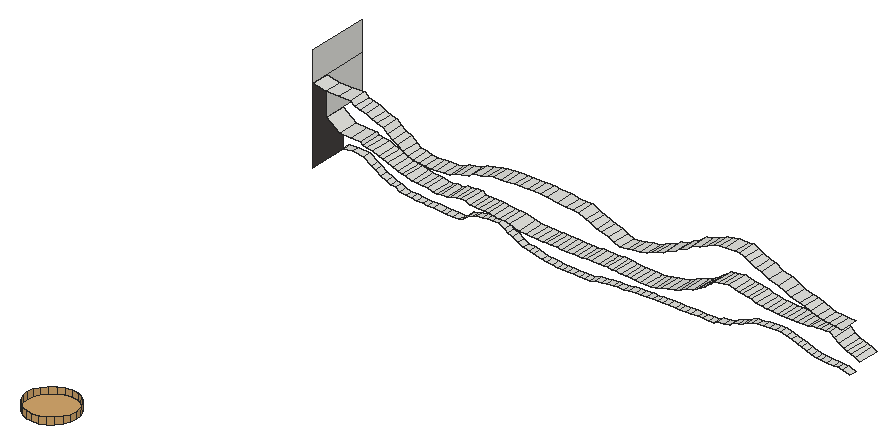
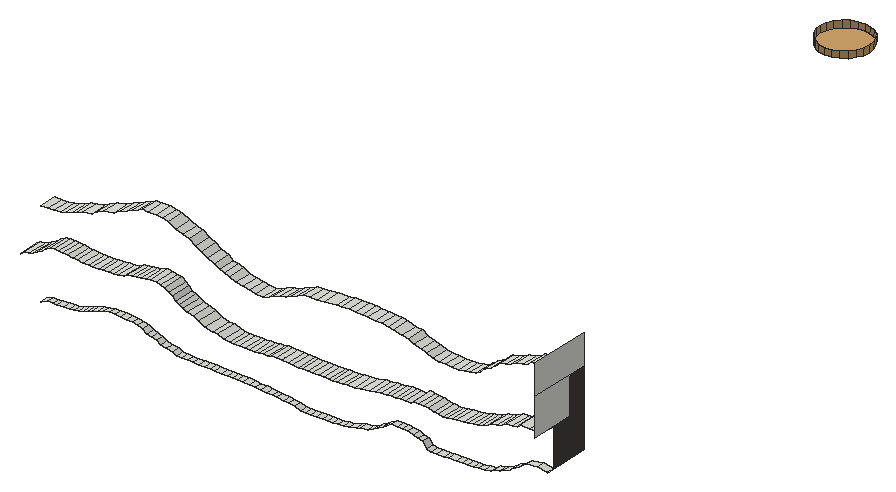
# SketchUp Ruby script. Lengths in inches.
U = 1.inch
M = Sketchup.active_model
def pt(a) = Geom::Point3d.new(a.map { |v| v * U })
def face(e, loops, mat)
  f = e.add_face(loops[0].map { |a| pt(a) })
  loops[1..].each { |l| e.add_face(l.map { |a| pt(a) }).erase! }
  f.material = f.back_material = mat if mat
  f
end
# faces: each face lists its corners as indices into pts; further lists are holes
def faces(e, pts, list, mat = nil) = list.each { |f| face(e, (f[0].is_a?(Array) ? f : [f]).map { |l| l.map { |i| pts[i] } }, mat) }
# xy, xz, yz: faces in a plane at the given z, y or x. An outline is a flat list of corners, or four numbers for a rectangle; further outlines are holes
def ring(l) = l.size == 4 ? [[l[0], l[1]], [l[2], l[1]], [l[2], l[3]], [l[0], l[3]]] : l.each_slice(2).to_a
def flat(e, list, mat, &to3) = list.each { |f| face(e, (f[0].is_a?(Array) ? f : [f]).map { |l| ring(l).map { |u, v| to3.(u, v) } }, mat) }
def xy(e, z, list, mat = nil) = flat(e, list, mat) { |x, y| [x, y, z] }
def xz(e, y, list, mat = nil) = flat(e, list, mat) { |x, z| [x, y, z] }
def yz(e, x, list, mat = nil) = flat(e, list, mat) { |y, z| [x, y, z] }
def lines(e, pts, list) = list.each { |a, b| e.add_line(pt(pts[a]), pt(pts[b])) }
# prism: a flat outline (further loops are holes) pulled along v
def prism(e, loops, v, mat = nil)
  f = face(e, loops, mat); d = Geom::Vector3d.new(v.map { |x| x * U })
  f.pushpull(f.normal.samedirection?(d) ? d.length : -d.length)
end
def box(e, o, s, mat = nil) = prism(e, [[o, [o[0] + s[0], o[1], o[2]], [o[0] + s[0], o[1] + s[1], o[2]], [o[0], o[1] + s[1], o[2]]]], [0, 0, s[2]], mat)
def at(x, y, z, deg = 0) = Geom::Transformation.translation(pt([x, y, z])) * Geom::Transformation.rotation(ORIGIN, Z_AXIS, deg.degrees)
def axes(o, x, y, z) = Geom::Transformation.new([*x, 0, *y, 0, *z, 0, *pt(o).to_a, 1])
def part(name) = M.definitions.add(name)
# library, detail: a bought-in or finely detailed component or shape, given as its bounding box
def library(name, o, s) = part(name).tap { |d| box(d.entities, o, s) }
def detail(e, o, s) = box(e.add_group.entities, o, s)
def put(e, d, t, mat = nil) = e.add_instance(d, t).tap { |i| i.material = mat if mat }
def group(e, t, mat = nil) = e.add_group.tap { |g| g.transformation = t; g.material = mat if mat }.entities
root = M.entities
M.materials.add("[Field Square Tile]").color = [211, 167, 108]
M.materials.add("[Granite Tile]1").color = [68, 65, 63]
xy(root,237.65,[[1160.83,565.74,1161.52,566.68],[1161.52,565.74,1162.14,566.68]])
xy(root,238.33,[[1169.93,565.74,1170.48,566.68],[1170.48,565.74,1171.16,566.68]])
xy(root,238.34,[[1171.84,565.74,1172.77,566.68],[1172.77,565.74,1173.26,566.68],[1173.26,565.74,1174.02,566.68],[1174.02,565.74,1174.65,566.68],[1174.65,565.74,1175.4,566.68],
  [1175.4,565.74,1176.02,566.68],[1176.02,565.74,1176.79,566.68],[1176.79,565.74,1177.41,566.68]])
xy(root,241.52,[[1131.53,561.05,1131.59,566.68]])
xy(root,241.68,[[1162.03,563.18,1162.62,565.74]])
xy(root,241.75,[[1164.38,563.18,1165.25,565.74],[1165.25,563.18,1165.87,565.74],[1165.87,563.18,1166.38,565.74]])
xy(root,250.6875,[[1151.85,492.27,1151.06,492.375,1150.32,492.68,1149.68,493.17,1149.2,493.8,1148.89,494.54,1148.79,495.33,1148.89,496.125,1149.2,496.86,1149.68,497.5,1150.32,497.98,1151.06,498.29,1151.85,498.39,1152.64,498.29,1153.38,497.98,1154.01,497.5,1154.5,496.86,1154.81,496.125,1154.91,495.33,1154.81,494.54,1154.5,493.8,1154.01,493.17,1153.38,492.68,1152.64,492.375]],"[Field Square Tile]")
xz(root,561.05,[[1131.53,241.52,1131.59,251.5]])
yz(root,1131.59,[[563.18,246.2,568.68,250.88],[561.05,250.88,568.68,254.5]])
yz(root,1131.59,[[561.05,241.52,565.74,241.52,565.74,246.2,563.18,246.2,563.18,250.88,561.05,250.88]],"[Granite Tile]1")
p = [[1162.14,565.74,237.65],[1162.14,566.68,237.65],[1162.81,566.68,237.89],[1162.81,565.74,237.89],[1157.47,565.74,237.76],[1157.47,566.68,237.76],
  [1158.18,566.68,237.71],[1158.18,565.74,237.71],[1158.79,566.68,237.68],[1158.79,565.74,237.68],[1159.39,566.68,237.67],[1159.39,565.74,237.67],
  [1160.14,566.68,237.66],[1160.14,565.74,237.66],[1160.83,566.68,237.65],[1160.83,565.74,237.65],[1156.12,565.74,237.9],[1156.12,566.68,237.9],
  [1156.78,566.68,237.82],[1156.78,565.74,237.82],[1155.18,565.74,238.21],[1155.18,566.68,238.21],[1163.57,566.68,237.94],[1163.57,565.74,237.94],
  [1164.1875,566.68,237.98],[1164.1875,565.74,237.98],[1165.04,566.68,238.1],[1165.04,565.74,238.1],[1165.59,566.68,238.13],[1165.59,565.74,238.13],
  [1166.35,566.68,238.15],[1166.35,565.74,238.15],[1154.71,565.74,238.31],[1154.71,566.68,238.31],[1166.98,566.68,238.26],[1166.98,565.74,238.26],
  [1153.8,565.74,238.43],[1153.8,566.68,238.43],[1167.73,566.68,238.28],[1167.73,565.74,238.28],[1168.36,566.68,238.3],[1168.36,565.74,238.3],
  [1169.21,566.68,238.32],[1169.21,565.74,238.32],[1169.93,566.68,238.33],[1169.93,565.74,238.33],[1171.16,565.74,238.33],[1171.16,566.68,238.33],
  [1171.84,566.68,238.34],[1171.84,565.74,238.34],[1177.41,565.74,238.34],[1177.41,566.68,238.34],[1177.92,566.68,238.59],[1177.92,565.74,238.59],
  [1153.15,565.74,238.74],[1153.15,566.68,238.74],[1193.44,565.74,238.78],[1193.44,566.68,238.78],[1194.22,566.68,238.43],[1194.22,565.74,238.43],
  [1178.74,566.68,238.72],[1178.74,565.74,238.72],[1152.57,565.74,239.11],[1152.57,566.68,239.11],[1179.43,566.68,238.86],[1179.43,565.74,238.86],
  [1142.78,565.74,238.92],[1142.78,566.68,238.92],[1143.82,566.68,238.82],[1143.82,565.74,238.82],[1144.33,566.68,238.8],[1144.33,565.74,238.8],
  [1145.2,566.68,238.79],[1145.2,565.74,238.79],[1145.94,566.68,238.77],[1145.94,565.74,238.77],[1146.47,566.68,238.9375],[1146.47,565.74,238.9375],
  [1190.72,565.74,238.875],[1190.72,566.68,238.875],[1191.47,566.68,238.83],[1191.47,565.74,238.83],[1192.23,566.68,238.8],[1192.23,565.74,238.8],
  [1192.77,566.68,238.79],[1192.77,565.74,238.79],[1140.69,565.74,238.97],[1140.69,566.68,238.97],[1141.39,566.68,238.94],[1141.39,565.74,238.94],
  [1142.09,566.68,238.93],[1142.09,565.74,238.93],[1147.03,566.68,239.55],[1147.03,565.74,239.55],[1179.94,566.68,239.18],[1179.94,565.74,239.18],
  [1189.57,565.74,239.04],[1189.57,566.68,239.04],[1190.15,566.68,238.94],[1190.15,565.74,238.94],[1139.32,565.74,239.09],[1139.32,566.68,239.09],
  [1140.01,566.68,239.03],[1140.01,565.74,239.03],[1188.91,565.74,239.29],[1188.91,566.68,239.29],[1138.54,565.74,239.19],[1138.54,566.68,239.19],
  [1151.99,565.74,239.38],[1151.99,566.68,239.38],[1138.03,565.74,239.52],[1138.03,566.68,239.52],[1180.53,566.68,239.35],[1180.53,565.74,239.35],
  [1188.33,565.74,239.53],[1188.33,566.68,239.53],[1151.53,565.74,239.71],[1151.53,566.68,239.71],[1181.09,566.68,239.52],[1181.09,565.74,239.52],
  [1137.47,565.74,239.64],[1137.47,566.68,239.64],[1181.64,566.68,239.85],[1181.64,565.74,239.85],[1187.8,565.74,239.7],[1187.8,566.68,239.7],
  [1137.02,565.74,239.86],[1137.02,566.68,239.86],[1147.61,566.68,239.69],[1147.61,565.74,239.69],[1148.16,566.68,239.88],[1148.16,565.74,239.88],
  [1150.83,565.74,240.11],[1150.83,566.68,240.11],[1187.11,565.74,239.92],[1187.11,566.68,239.92],[1182.28,566.68,240.03],[1182.28,565.74,240.03],
  [1136.23,565.74,240.2],[1136.23,566.68,240.2],[1148.89,566.68,239.99],[1148.89,565.74,239.99],[1186.48,565.74,240.11],[1186.48,566.68,240.11],
  [1149.48,566.68,240.05],[1149.48,565.74,240.05],[1150.14,566.68,240.09],[1150.14,565.74,240.09],[1182.9375,566.68,240.12],[1182.9375,565.74,240.12],
  [1183.61,566.68,240.19],[1183.61,565.74,240.19],[1185.7,565.74,240.27],[1185.7,566.68,240.27],[1135.63,565.74,240.59],[1135.63,566.68,240.59],
  [1184.375,566.68,240.23],[1184.375,565.74,240.23],[1185.08,566.68,240.25],[1185.08,565.74,240.25],[1135.09,565.74,240.85],[1135.09,566.68,240.85],
  [1134.07,565.74,241.55],[1134.07,566.68,241.55],[1168.01,563.18,241.57],[1168.01,565.74,241.57],[1168.55,565.74,241.53],[1168.55,563.18,241.53],
  [1169.17,565.74,241.51],[1169.17,563.18,241.51],[1169.72,565.74,241.49],[1169.72,563.18,241.49],[1170.42,565.74,241.48],[1170.42,563.18,241.48],
  [1171.08,565.74,241.47],[1171.08,563.18,241.47],[1171.65,565.74,241.46],[1171.65,563.18,241.46],[1172.36,565.74,241.6],[1172.36,563.18,241.6],
  [1131.59,565.74,241.52],[1131.59,566.68,241.52],[1132.8,566.68,241.69],[1132.8,565.74,241.69],[1167.4,563.18,241.66],[1167.4,565.74,241.66],
  [1173.09,565.74,241.85],[1173.09,563.18,241.85],[1158.37,563.18,241.75],[1158.37,565.74,241.75],[1158.82,565.74,241.74],[1158.82,563.18,241.74],
  [1159.37,565.74,241.72],[1159.37,563.18,241.72],[1160,565.74,241.71],[1160,563.18,241.71],[1160.63,565.74,241.7],[1160.63,563.18,241.7],
  [1161.36,565.74,241.69],[1161.36,563.18,241.69],[1162.03,565.74,241.68],[1162.03,563.18,241.68],[1162.62,563.18,241.68],[1162.62,565.74,241.68],
  [1163.11,565.74,241.67],[1163.11,563.18,241.67],[1163.8125,565.74,241.74],[1163.8125,563.18,241.74],[1164.38,565.74,241.75],[1164.38,563.18,241.75],
  [1166.38,563.18,241.75],[1166.38,565.74,241.75],[1166.87,565.74,241.67],[1166.87,563.18,241.67],[1156.18,563.18,241.89],[1156.18,565.74,241.89],
  [1157,565.74,241.83],[1157,563.18,241.83],[1157.6,565.74,241.78],[1157.6,563.18,241.78],[1173.76,565.74,241.91],[1173.76,563.18,241.91],
  [1155.41,563.18,241.96],[1155.41,565.74,241.96],[1174.66,565.74,242.1],[1174.66,563.18,242.1],[1154.24,563.18,242.24],[1154.24,565.74,242.24],
  [1175.43,565.74,242.46],[1175.43,563.18,242.46],[1153.57,563.18,242.34],[1153.57,565.74,242.34],[1197.04,563.18,242.51],[1197.04,565.74,242.51],
  [1197.55,565.74,242.21],[1197.55,563.18,242.21],[1152.91,563.18,242.38],[1152.91,565.74,242.38],[1152.25,563.18,242.48],[1152.25,565.74,242.48],
  [1144.07,563.18,242.68],[1144.07,565.74,242.68],[1144.74,565.74,242.51],[1144.74,563.18,242.51],[1145.26,565.74,242.46],[1145.26,563.18,242.46],
  [1145.8,565.74,242.58],[1145.8,563.18,242.58],[1151.61,563.18,242.57],[1151.61,565.74,242.57],[1176.13,565.74,242.78],[1176.13,563.18,242.78],
  [1196.45,563.18,242.68],[1196.45,565.74,242.68],[1146.43,565.74,242.57],[1146.43,563.18,242.57],[1147.06,565.74,242.81],[1147.06,563.18,242.81],
  [1148.83,563.18,242.92],[1148.83,565.74,242.92],[1149.26,565.74,242.625],[1149.26,563.18,242.625],[1149.87,565.74,242.65],[1149.87,563.18,242.65],
  [1150.42,565.74,242.62],[1150.42,563.18,242.62],[1151.05,565.74,242.58],[1151.05,563.18,242.58],[1142.72,563.18,242.78],[1142.72,565.74,242.78],
  [1143.53,565.74,242.73],[1143.53,563.18,242.73],[1195.95,563.18,242.875],[1195.95,565.74,242.875],[1141.42,563.18,243.06],[1141.42,565.74,243.06],
  [1142.14,565.74,242.85],[1142.14,563.18,242.85],[1147.63,565.74,242.86],[1147.63,563.18,242.86],[1176.9,565.74,242.97],[1176.9,563.18,242.97],
  [1148.19,565.74,242.89],[1148.19,563.18,242.89],[1195.56,563.18,243.09],[1195.56,565.74,243.09],[1177.43,565.74,243.23],[1177.43,563.18,243.23],
  [1140.35,563.18,243.3],[1140.35,565.74,243.3],[1140.9375,565.74,243.14],[1140.9375,563.18,243.14],[1194.95,563.18,243.43],[1194.95,565.74,243.43],
  [1177.83,565.74,243.48],[1177.83,563.18,243.48],[1139.71,563.18,243.48],[1139.71,565.74,243.48],[1194.41,563.18,243.8],[1194.41,565.74,243.8],
  [1139.19,563.18,243.79],[1139.19,565.74,243.79],[1178.35,565.74,243.72],[1178.35,563.18,243.72],[1178.6875,565.74,244.12],[1178.6875,563.18,244.12],
  [1138.53,563.18,243.95],[1138.53,565.74,243.95],[1193.81,563.18,244.18],[1193.81,565.74,244.18],[1138.01,563.18,244.11],[1138.01,565.74,244.11],
  [1186.63,563.18,243.99],[1186.63,565.74,243.99],[1187.35,565.74,243.95],[1187.35,563.18,243.95],[1187.85,565.74,243.93],[1187.85,563.18,243.93],
  [1188.54,565.74,243.91],[1188.54,563.18,243.91],[1189.11,565.74,243.89],[1189.11,563.18,243.89],[1189.81,565.74,243.88],[1189.81,563.18,243.88],
  [1190.46,565.74,243.94],[1190.46,563.18,243.94],[1191.1,565.74,243.95],[1191.1,563.18,243.95],[1191.66,565.74,244.1],[1191.66,563.18,244.1],
  [1185.45,563.18,244.11],[1185.45,565.74,244.11],[1186.01,565.74,244.04],[1186.01,563.18,244.04],[1137.34,563.18,244.41],[1137.34,565.74,244.41],
  [1179.16,565.74,244.39],[1179.16,563.18,244.39],[1184.7,563.18,244.25],[1184.7,565.74,244.25],[1192.29,565.74,244.13],[1192.29,563.18,244.13],
  [1192.77,565.74,244.15],[1192.77,563.18,244.15],[1193.29,565.74,244.17],[1193.29,563.18,244.17],[1184.24,563.18,244.51],[1184.24,565.74,244.51],
  [1136.58,563.18,244.54],[1136.58,565.74,244.54],[1179.64,565.74,244.73],[1179.64,563.18,244.73],[1136.02,563.18,244.61],[1136.02,565.74,244.61],
  [1183.09,563.18,244.67],[1183.09,565.74,244.67],[1183.7,565.74,244.55],[1183.7,563.18,244.55],[1135.8,563.18,244.92],[1135.8,565.74,244.92],
  [1180.125,565.74,244.87],[1180.125,563.18,244.87],[1182.04,563.18,244.81],[1182.04,565.74,244.81],[1182.61,565.74,244.7],[1182.61,563.18,244.7],
  [1181.39,563.18,245.01],[1181.39,565.74,245.01],[1133.16,563.18,244.96],[1133.16,565.74,244.96],[1134.55,565.74,244.9375],[1134.55,563.18,244.9375],
  [1180.71,565.74,244.95],[1180.71,563.18,244.95],[1131.59,563.18,246.2],[1131.59,565.74,246.2],[1168.84,561.05,246.35],[1168.84,563.18,246.35],
  [1169.61,563.18,246.05],[1169.61,561.05,246.05],[1170.51,563.18,246.13],[1170.51,561.05,246.13],[1171.22,563.18,246.29],[1171.22,561.05,246.29],
  [1172.02,563.18,246.41],[1172.02,561.05,246.41],[1168.23,561.05,246.66],[1168.23,563.18,246.66],[1172.93,563.18,246.55],[1172.93,561.05,246.55],
  [1144.65,561.05,246.62],[1144.65,563.18,246.62],[1145.39,563.18,246.54],[1145.39,561.05,246.54],[1146.17,563.18,246.51],[1146.17,561.05,246.51],
  [1146.95,563.18,246.58],[1146.95,561.05,246.58],[1196.14,561.05,246.59],[1196.14,563.18,246.59],[1197.03,563.18,246.55],[1197.03,561.05,246.55],
  [1143.99,561.05,246.73],[1143.99,563.18,246.73],[1147.75,563.18,246.59],[1147.75,561.05,246.59],[1148.55,563.18,246.69],[1148.55,561.05,246.69],
  [1173.66,563.18,246.92],[1173.66,561.05,246.92],[1195.43,561.05,246.66],[1195.43,563.18,246.66],[1143.27,561.05,246.88],[1143.27,563.18,246.88],
  [1149.26,563.18,247.03],[1149.26,561.05,247.03],[1167.375,561.05,246.94],[1167.375,563.18,246.94],[1194.64,561.05,246.75],[1194.64,563.18,246.75],
  [1193.95,561.05,246.95],[1193.95,563.18,246.95],[1142.72,561.05,247.25],[1142.72,563.18,247.25],[1166.69,561.05,247.08],[1166.69,563.18,247.08],
  [1174.27,563.18,247.12],[1174.27,561.05,247.12],[1149.95,563.18,247.2],[1149.95,561.05,247.2],[1193.14,561.05,247.25],[1193.14,563.18,247.25],
  [1166.01,561.05,247.46],[1166.01,563.18,247.46],[1174.95,563.18,247.31],[1174.95,561.05,247.31],[1150.92,563.18,247.39],[1150.92,561.05,247.39],
  [1192.46,561.05,247.53],[1192.46,563.18,247.53],[1142.08,561.05,247.72],[1142.08,563.18,247.72],[1175.52,563.18,247.71],[1175.52,561.05,247.71],
  [1151.55,563.18,247.78],[1151.55,561.05,247.78],[1165.38,561.05,247.66],[1165.38,563.18,247.66],[1191.88,561.05,247.66],[1191.88,563.18,247.66],
  [1141.43,561.05,248.07],[1141.43,563.18,248.07],[1164.54,561.05,248.08],[1164.54,563.18,248.08],[1176.45,563.18,248.03],[1176.45,561.05,248.03],
  [1190.75,561.05,247.9],[1190.75,563.18,247.9],[1152.33,563.18,247.89],[1152.33,561.05,247.89],[1153.33,563.18,248.18],[1153.33,561.05,248.18],
  [1190.15,561.05,248.26],[1190.15,563.18,248.26],[1177.16,563.18,248.46],[1177.16,561.05,248.46],[1140.8,561.05,248.51],[1140.8,563.18,248.51],
  [1162.92,561.05,248.15],[1162.92,563.18,248.15],[1163.74,563.18,248.11],[1163.74,561.05,248.11],[1153.97,563.18,248.29],[1153.97,561.05,248.29],
  [1161.89,561.05,248.28],[1161.89,563.18,248.28],[1154.86,563.18,248.35],[1154.86,561.05,248.35],[1160.49,561.05,248.39],[1160.49,563.18,248.39],
  [1189.24,561.05,248.69],[1189.24,563.18,248.69],[1155.59,563.18,248.4],[1155.59,561.05,248.4],[1156.58,563.18,248.4375],[1156.58,561.05,248.4375],
  [1157.24,563.18,248.46],[1157.24,561.05,248.46],[1159.76,561.05,248.49],[1159.76,563.18,248.49],[1140.31,561.05,249.01],[1140.31,563.18,249.01],
  [1158.13,563.18,248.47],[1158.13,561.05,248.47],[1158.87,563.18,248.48],[1158.87,561.05,248.48],[1177.94,563.18,248.82],[1177.94,561.05,248.82],
  [1188.02,561.05,248.95],[1188.02,563.18,248.95],[1178.66,563.18,249.37],[1178.66,561.05,249.37],[1187.13,561.05,249.46],[1187.13,563.18,249.46],
  [1139.54,561.05,249.2],[1139.54,563.18,249.2],[1138.87,561.05,249.41],[1138.87,563.18,249.41],[1138.2,561.05,249.8],[1138.2,563.18,249.8],
  [1179.45,563.18,249.5625],[1179.45,561.05,249.5625],[1186.37,561.05,249.68],[1186.37,563.18,249.68],[1180.35,563.18,249.9],[1180.35,561.05,249.9],
  [1185.71,561.05,250.0625],[1185.71,563.18,250.0625],[1137.4,561.05,249.97],[1137.4,563.18,249.97],[1181.27,563.18,250.35],[1181.27,561.05,250.35],
  [1136.79,561.05,250.15],[1136.79,563.18,250.15],[1136.26,561.05,250.55],[1136.26,563.18,250.55],[1185.02,561.05,250.32],[1185.02,563.18,250.32],
  [1181.93,563.18,250.49],[1181.93,561.05,250.49],[1184.4,561.05,250.61],[1184.4,563.18,250.61],[1131.59,561.05,250.88],[1131.59,563.18,250.88],
  [1133.18,563.18,250.53],[1133.18,561.05,250.53],[1134.8,563.18,250.54],[1134.8,561.05,250.54],[1182.74,563.18,250.6],[1182.74,561.05,250.6],
  [1183.76,563.18,250.58],[1183.76,561.05,250.58],[1151.85,492.27,251.5],[1151.06,492.375,251.5],[1151.06,492.375,250.6875],[1151.85,492.27,250.6875],
  [1152.64,492.375,251.5],[1152.64,492.375,250.6875],[1150.32,492.68,251.5],[1150.32,492.68,250.6875],[1153.38,492.68,251.5],[1153.38,492.68,250.6875],
  [1149.68,493.17,251.5],[1149.68,493.17,250.6875],[1154.01,493.17,251.5],[1154.01,493.17,250.6875],[1149.2,493.8,251.5],[1149.2,493.8,250.6875],
  [1154.5,493.8,251.5],[1154.5,493.8,250.6875],[1148.89,494.54,251.5],[1148.89,494.54,250.6875],[1154.81,494.54,251.5],[1154.81,494.54,250.6875],
  [1148.79,495.33,251.5],[1148.79,495.33,250.6875],[1154.91,495.33,251.5],[1154.91,495.33,250.6875],[1148.89,496.125,251.5],[1148.89,496.125,250.6875],
  [1154.81,496.125,251.5],[1154.81,496.125,250.6875],[1149.2,496.86,251.5],[1149.2,496.86,250.6875],[1154.5,496.86,251.5],[1154.5,496.86,250.6875],
  [1149.68,497.5,251.5],[1149.68,497.5,250.6875],[1154.01,497.5,251.5],[1154.01,497.5,250.6875],[1150.32,497.98,251.5],[1150.32,497.98,250.6875],
  [1153.38,497.98,251.5],[1153.38,497.98,250.6875],[1151.06,498.29,251.5],[1151.06,498.29,250.6875],[1152.64,498.29,251.5],[1152.64,498.29,250.6875],
  [1151.85,498.39,251.5],[1151.85,498.39,250.6875]]
faces(root,p,[[0,1,2,3],[4,5,6,7],[7,6,8,9],[9,8,10,11],[11,10,12,13],[13,12,14,15],[16,17,18,19],[19,18,5,4],
  [20,21,17,16],[3,2,22,23],[23,22,24,25],[25,24,26,27],[27,26,28,29],[29,28,30,31],[32,33,21,20],[31,30,34,35],
  [36,37,33,32],[35,34,38,39],[39,38,40,41],[41,40,42,43],[43,42,44,45],[46,47,48,49],[50,51,52,53],[54,55,37,36],
  [56,57,58,59],[53,52,60,61],[62,63,55,54],[61,60,64,65],[66,67,68,69],[69,68,70,71],[71,70,72,73],[73,72,74,75],
  [75,74,76,77],[78,79,80,81],[81,80,82,83],[83,82,84,85],[85,84,57,56],[86,87,88,89],[89,88,90,91],[91,90,67,66],
  [77,76,92,93],[65,64,94,95],[96,97,98,99],[99,98,79,78],[100,101,102,103],[103,102,87,86],[104,105,97,96],[106,107,101,100],
  [108,109,63,62],[110,111,107,106],[95,94,112,113],[114,115,105,104],[116,117,109,108],[113,112,118,119],[120,121,111,110],[119,118,122,123],
  [124,125,115,114],[126,127,121,120],[93,92,128,129],[129,128,130,131],[132,133,117,116],[134,135,125,124],[123,122,136,137],[138,139,127,126],
  [131,130,140,141],[142,143,135,134],[141,140,144,145],[145,144,146,147],[137,136,148,149],[147,146,133,132],[149,148,150,151],[152,153,143,142],
  [154,155,139,138],[151,150,156,157],[157,156,158,159],[159,158,153,152],[160,161,155,154],[162,163,161,160],[164,165,166,167],[167,166,168,169],
  [169,168,170,171],[171,170,172,173],[173,172,174,175],[175,174,176,177],[177,176,178,179],[180,181,182,183],[184,185,165,164],[179,178,186,187],
  [183,182,163,162],[188,189,190,191],[191,190,192,193],[193,192,194,195],[195,194,196,197],[197,196,198,199],[199,198,200,201],[202,203,204,205],
  [205,204,206,207],[207,206,208,209],[210,211,212,213],[213,212,185,184],[214,215,216,217],[217,216,218,219],[219,218,189,188],[187,186,220,221],
  [222,223,215,214],[221,220,224,225],[226,227,223,222],[225,224,228,229],[230,231,227,226],[232,233,234,235],[236,237,231,230],[238,239,237,236],
  [240,241,242,243],[243,242,244,245],[245,244,246,247],[248,249,239,238],[229,228,250,251],[252,253,233,232],[247,246,254,255],[255,254,256,257],
  [258,259,260,261],[261,260,262,263],[263,262,264,265],[265,264,266,267],[267,266,249,248],[268,269,270,271],[271,270,241,240],[272,273,253,252],
  [274,275,276,277],[277,276,269,268],[257,256,278,279],[251,250,280,281],[279,278,282,283],[283,282,259,258],[284,285,273,272],[281,280,286,287],
  [288,289,290,291],[291,290,275,274],[292,293,285,284],[287,286,294,295],[296,297,289,288],[298,299,293,292],[300,301,297,296],[295,294,302,303],
  [303,302,304,305],[306,307,301,300],[308,309,299,298],[310,311,307,306],[312,313,314,315],[315,314,316,317],[317,316,318,319],[319,318,320,321],
  [321,320,322,323],[323,322,324,325],[325,324,326,327],[327,326,328,329],[330,331,332,333],[333,332,313,312],[334,335,311,310],[305,304,336,337],
  [338,339,331,330],[329,328,340,341],[341,340,342,343],[343,342,344,345],[345,344,309,308],[346,347,339,338],[348,349,335,334],[337,336,350,351],
  [352,353,349,348],[354,355,356,357],[357,356,347,346],[358,359,353,352],[351,350,360,361],[362,363,364,365],[365,364,355,354],[366,367,363,362],
  [368,369,370,371],[371,370,359,358],[361,360,372,373],[373,372,367,366],[374,375,369,368],[376,377,378,379],[379,378,380,381],[381,380,382,383],
  [383,382,384,385],[386,387,377,376],[385,384,388,389],[390,391,392,393],[393,392,394,395],[395,394,396,397],[398,399,400,401],[402,403,391,390],
  [397,396,404,405],[405,404,406,407],[389,388,408,409],[410,411,399,398],[412,413,403,402],[407,406,414,415],[416,417,387,386],[418,419,411,410],
  [420,421,419,418],[422,423,413,412],[424,425,417,416],[409,408,426,427],[415,414,428,429],[430,431,421,420],[432,433,425,424],[427,426,434,435],
  [429,428,436,437],[438,439,431,430],[440,441,423,422],[435,434,442,443],[437,436,444,445],[446,447,433,432],[448,449,439,438],[450,451,441,440],
  [452,453,447,446],[443,442,454,455],[456,457,449,448],[445,444,458,459],[459,458,460,461],[462,463,457,456],[455,454,464,465],[466,467,451,450],
  [468,469,470,471],[471,470,453,452],[461,460,472,473],[474,475,469,468],[473,472,476,477],[478,479,475,474],[480,481,463,462],[477,476,482,483],
  [483,482,484,485],[485,484,486,487],[488,489,479,478],[490,491,467,466],[487,486,492,493],[493,492,494,495],[495,494,489,488],[465,464,496,497],
  [498,499,481,480],[497,496,500,501],[502,503,499,498],[504,505,491,490],[506,507,505,504],[508,509,507,506],[501,500,510,511],[512,513,503,502],
  [511,510,514,515],[516,517,513,512],[518,519,509,508],[515,514,520,521],[522,523,519,518],[524,525,523,522],[526,527,517,516],[521,520,528,529],
  [530,531,527,526],[532,533,534,535],[535,534,536,537],[537,536,525,524],[529,528,538,539],[539,538,540,541],[541,540,531,530]])
faces(root,p,[[542,543,544,545],[546,542,545,547],[543,548,549,544],[550,546,547,551],[548,552,553,549],[554,550,551,555],[552,556,557,553],[558,554,555,559],
  [556,560,561,557],[562,558,559,563],[560,564,565,561],[566,562,563,567],[564,568,569,565],[570,566,567,571],[568,572,573,569],[574,570,571,575],
  [572,576,577,573],[578,574,575,579],[576,580,581,577],[582,578,579,583],[580,584,585,581],[586,582,583,587],[584,588,589,585],[588,586,587,589]],"[Field Square Tile]")
